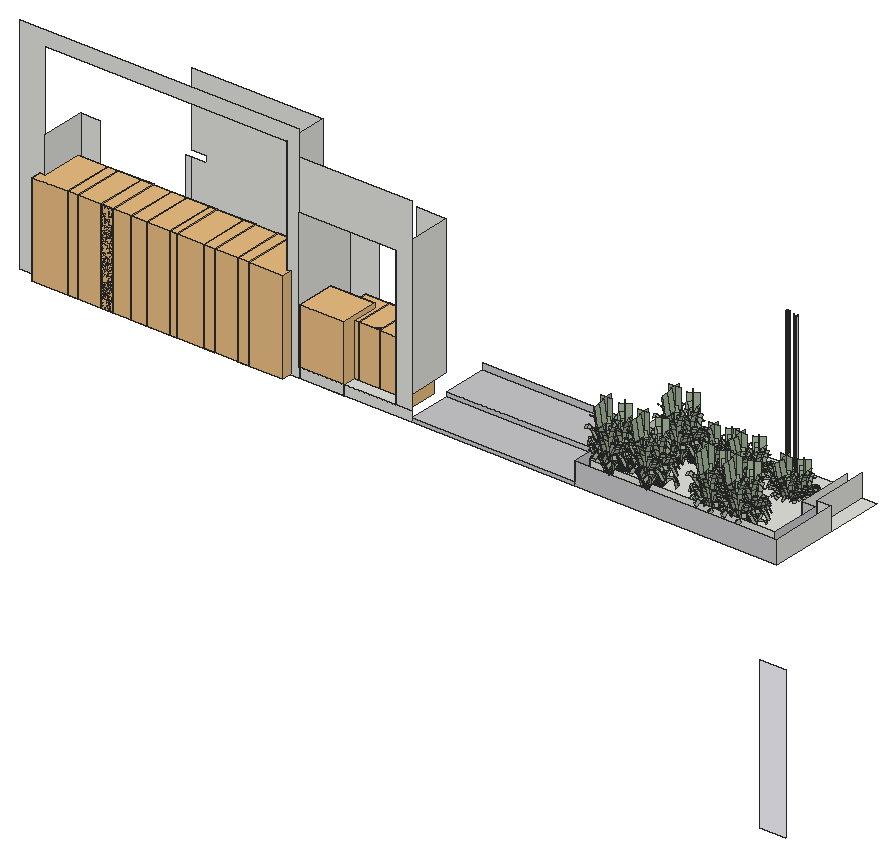
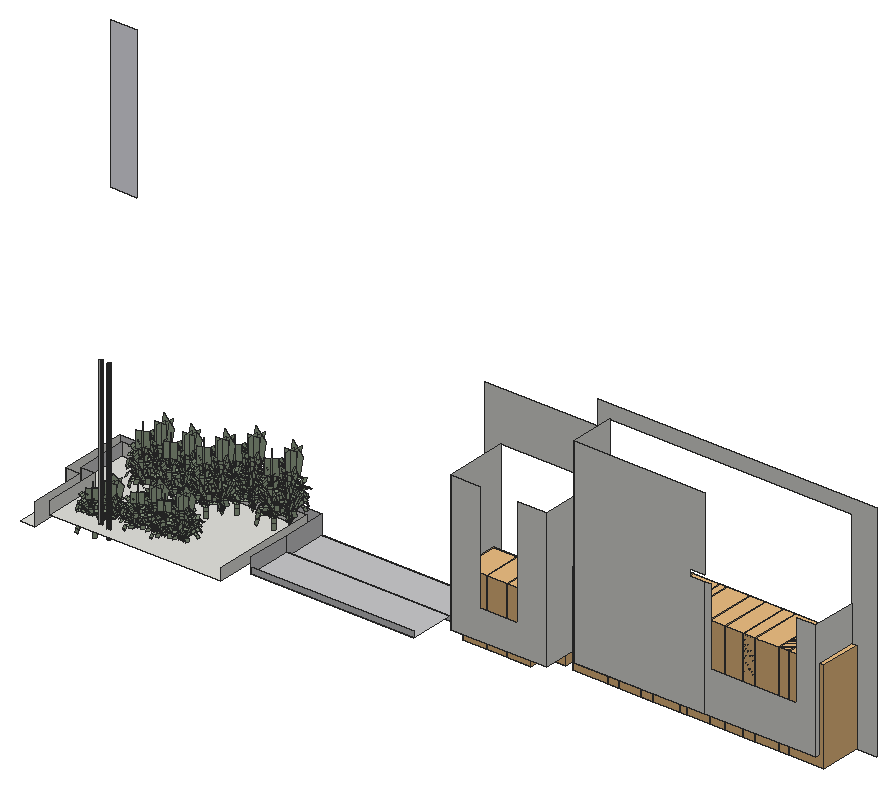
# SketchUp Ruby script. Lengths in inches.
U = 1.inch
M = Sketchup.active_model
def pt(a) = Geom::Point3d.new(a.map { |v| v * U })
def face(e, loops, mat)
  f = e.add_face(loops[0].map { |a| pt(a) })
  loops[1..].each { |l| e.add_face(l.map { |a| pt(a) }).erase! }
  f.material = f.back_material = mat if mat
  f
end
# faces: each face lists its corners as indices into pts; further lists are holes
def faces(e, pts, list, mat = nil) = list.each { |f| face(e, (f[0].is_a?(Array) ? f : [f]).map { |l| l.map { |i| pts[i] } }, mat) }
# xy, xz, yz: faces in a plane at the given z, y or x. An outline is a flat list of corners, or four numbers for a rectangle; further outlines are holes
def ring(l) = l.size == 4 ? [[l[0], l[1]], [l[2], l[1]], [l[2], l[3]], [l[0], l[3]]] : l.each_slice(2).to_a
def flat(e, list, mat, &to3) = list.each { |f| face(e, (f[0].is_a?(Array) ? f : [f]).map { |l| ring(l).map { |u, v| to3.(u, v) } }, mat) }
def xy(e, z, list, mat = nil) = flat(e, list, mat) { |x, y| [x, y, z] }
def xz(e, y, list, mat = nil) = flat(e, list, mat) { |x, z| [x, y, z] }
def yz(e, x, list, mat = nil) = flat(e, list, mat) { |y, z| [x, y, z] }
def lines(e, pts, list) = list.each { |a, b| e.add_line(pt(pts[a]), pt(pts[b])) }
# prism: a flat outline (further loops are holes) pulled along v
def prism(e, loops, v, mat = nil)
  f = face(e, loops, mat); d = Geom::Vector3d.new(v.map { |x| x * U })
  f.pushpull(f.normal.samedirection?(d) ? d.length : -d.length)
end
def box(e, o, s, mat = nil) = prism(e, [[o, [o[0] + s[0], o[1], o[2]], [o[0] + s[0], o[1] + s[1], o[2]], [o[0], o[1] + s[1], o[2]]]], [0, 0, s[2]], mat)
def at(x, y, z, deg = 0) = Geom::Transformation.translation(pt([x, y, z])) * Geom::Transformation.rotation(ORIGIN, Z_AXIS, deg.degrees)
def axes(o, x, y, z) = Geom::Transformation.new([*x, 0, *y, 0, *z, 0, *pt(o).to_a, 1])
def part(name) = M.definitions.add(name)
# library, detail: a bought-in or finely detailed component or shape, given as its bounding box
def library(name, o, s) = part(name).tap { |d| box(d.entities, o, s) }
def detail(e, o, s) = box(e.add_group.entities, o, s)
def put(e, d, t, mat = nil) = e.add_instance(d, t).tap { |i| i.material = mat if mat }
def group(e, t, mat = nil) = e.add_group.tap { |g| g.transformation = t; g.material = mat if mat }.entities
root = M.entities
M.materials.add("[0117_GhostWhite]").color = [248, 248, 255]
M.materials.add("[Polished Concrete New]").color = [200, 200, 203]
M.materials.add("hymenocallis littoralis").color = [156, 172, 146]
c1 = part("Group\#856")
xy(c1.entities,7.38,[[0,0,5.5,15.91]],"hymenocallis littoralis")
p = [[5.5,28.78,0],[5.5,26.79,3.44],[0,26.79,3.44],[0,28.78,0],[0,23.75,6],[5.5,23.75,6],
  [0,15.91,7.38],[5.5,15.91,7.38]]
faces(c1.entities,p,[[0,1,2,3],[4,2,1,5],[6,4,5,7]],"hymenocallis littoralis")
c2 = part("Group\#854")
xy(c2.entities,7.38,[[0,0,5.5,15.91],[0,15.91,5.5,23.87]],"hymenocallis littoralis")
p = [[5.5,31.07,4.3],[5.5,27.74,6.47],[0,27.74,6.47],[0,31.07,4.3],[0,23.87,7.38],[5.5,23.87,7.38]]
faces(c2.entities,p,[[0,1,2,3],[4,2,1,5]],"hymenocallis littoralis")
c3 = part("Group\#857")
xy(c3.entities,7.38,[[0,0,5.6,15.91]],"hymenocallis littoralis")
p = [[5.6,28.78,0],[5.6,26.79,3.44],[0,26.79,3.44],[0,28.78,0],[0,23.75,6],[5.6,23.75,6],
  [0,15.91,7.38],[5.6,15.91,7.38]]
faces(c3.entities,p,[[0,1,2,3],[4,2,1,5],[6,4,5,7]],"hymenocallis littoralis")
c4 = part("Group\#855")
put(c4.entities,c2,axes([6.09,8.57,-0.52],[0.446,0.85617,0.26089],[-0.18444,-0.19731,0.96283],[0.87582,-0.47754,0.0699]))
put(c4.entities,c2,axes([6.29,7.28,-1.71],[0.37058,0.92707,-0.05667],[-0.32382,0.19004,0.99128],[0.87712,-0.32925,0.34964]))
put(c4.entities,c2,axes([11.04,16.14,-0.7],[1,0,0],[0,0.16628,1.02662],[0,-1.18456,0.19186]))
c5 = part("Group\#860")
put(c5.entities,c1,axes([24.57,32.05,-1.76],[0.9552,-0.22102,-0.19681],[0.4036,0.95545,0.88585],[-0.00568,-0.67859,0.7345]))
put(c5.entities,c1,axes([23.95,29.24,-2.4],[0,1,0],[-0.76041,0,0.64945],[0.64945,0,0.76041]))
put(c5.entities,c1,axes([24.22,24.72,-0.48],[-0.70711,0.70711,0],[-0.32757,-0.32757,0.80237],[0.61237,0.61237,0.5]))
put(c5.entities,c2,axes([20.66,37.22,-0.63],[1.12361,0.03262,0.39091],[-0.43499,0.29739,0.78777],[0.09852,-1.27434,0.37535]))
put(c5.entities,c1,axes([28.75,24.45,-2.4],[-1,0,0],[0,-0.76041,0.64945],[0,0.64945,0.76041]))
put(c5.entities,c3,axes([30.4,30.98,-3.7],[0.65676,-0.72002,0.22414],[0.55667,0.66341,0.5],[-0.50871,-0.20361,0.83652]))
put(c5.entities,c3,axes([32.41,29.61,-3.7],[0.04029,-0.97372,0.22414],[0.85287,0.15038,0.5],[-0.52057,0.17102,0.83652]))
put(c5.entities,c1,axes([31.89,25.85,-1.76],[-0.92056,0.33739,-0.19681],[-0.5186,-0.89824,0.88585],[0.08952,0.67268,0.7345]))
put(c5.entities,c1,axes([25.55,34.78,-0.48],[0.86603,0.5,0],[-0.25,0.43301,0.86603],[0.43301,-0.75,0.5]))
put(c5.entities,c3,axes([20.4,16.9375,-8.07],[-0.70711,0.70711,0],[-0.35754,-0.35754,0.65422],[1.3987,1.3987,1.52882]))
put(c5.entities,c1,axes([32.86,34.14,-0.48],[0.76604,-0.64279,0],[0.32139,0.38302,0.86603],[-0.55667,-0.66341,0.5]))
put(c5.entities,c1,axes([27.15,34.7,-0.1],[0.82472,-0.17528,-0.53769],[0.53769,0.53769,0.64945],[0.17528,-0.82472,0.53769]))
put(c5.entities,c1,axes([33.58,28.77,-2.4],[0,-1,0],[0.76041,0,0.64945],[-0.64945,0,0.76041]))
put(c5.entities,c1,axes([26.43,23.87,-2.81],[-0.75126,0.04415,0.65853],[0.53769,-0.53769,0.64945],[0.38276,0.84199,0.3802]))
put(c5.entities,c1,axes([28.78,23.98,-2.4],[-1,0,0],[0,-0.76041,0.64945],[0,0.64945,0.76041]))
put(c5.entities,c1,axes([25.39,25.38,-2.4],[-0.70711,0.70711,0],[-0.53769,-0.53769,0.64945],[0.45923,0.45923,0.76041]))
put(c5.entities,c1,axes([27.32,21.63,-0.1],[-0.45923,0.70711,-0.53769],[-0.76041,0,0.64945],[0.45923,0.70711,0.53769]))
put(c5.entities,c1,axes([25.17,27.625,-1.76],[0.56416,0.80187,-0.19681],[-0.66673,0.66673,0.80532],[0.62659,-0.26057,0.7345]))
put(c5.entities,c3,axes([27.59,27.04,-3.96],[-0.8993,-0.06127,0.43301],[0.2962,-0.8138,0.5],[0.32175,0.57791,0.75]))
put(c5.entities,c3,axes([26.98,24.5,-3.18],[-0.5,0.86603,0],[-0.75,-0.43301,0.5],[0.43301,0.25,0.86603]))
put(c5.entities,c3,axes([24.55,27.74,-3.7],[0.29517,0.92878,0.22414],[-0.85287,0.15038,0.5],[0.43068,-0.33875,0.83652]))
put(c5.entities,c3,axes([24.26,29.8,-3.18],[0.76604,0.64279,0],[-0.47317,0.5639,0.425],[0.32139,-0.38302,0.86603]))
put(c5.entities,c3,axes([25.98,32.46,-3.18],[1,0,0],[0,0.86603,0.5],[0,-0.5,0.86603]))
put(c5.entities,c1,axes([28.78,33.57,-2.4],[1,0,0],[0,0.76041,0.64945],[0,-0.64945,0.76041]))
put(c5.entities,c4,at(14.99,21.38,2.5))
put(c5.entities,c2,axes([34.63,26.34,-1.46],[-0.70089,-0.70877,0.07994],[0.4756,-0.38088,0.79293],[-0.53156,0.59378,0.60405]))
put(c5.entities,c2,axes([28.14,16.92,1.8125],[-1.19719,0.6912,0],[-0.09607,-0.16641,0.94244],[0.68444,1.18549,0.17613]))
put(c5.entities,c2,axes([31.5625,35.84,0.97],[0.66765,-1.1564,0.35779],[0.04445,0.30732,0.91033],[-1.20828,-0.64496,0.17012]))
put(c5.entities,c2,axes([38.94,22.51,0.89],[-0.97932,-0.67164,-0.05202],[0.27787,-0.41401,0.90999],[-0.85985,0.93577,0.32097]))
put(c5.entities,c2,axes([38.44,21.09,1.98],[-1.02864,-0.54856,0.2395],[0.33481,0.06999,0.88388],[-0.77261,1.08328,0.06417]))
put(c5.entities,c3,axes([35.02,30.51,-1.3],[-0.17365,-0.98481,0],[0.60224,-0.10619,0.79122],[-0.7792,0.13739,0.61153]))
put(c5.entities,c3,axes([29.41,22.33,-1.3],[-0.93969,0.34202,0],[-0.20915,-0.57465,0.79122],[0.27061,0.74351,0.61153]))
put(c5.entities,c2,axes([19.64,36,-1.62],[1.18194,0.09546,0.08234],[-0.14377,0.68823,0.76313],[0.21457,-1.1326,0.62386]))
put(c5.entities,c3,axes([24.25,24.14,-1.3],[-0.34202,0.93969,0],[-0.57465,-0.20915,0.79122],[0.74351,0.27061,0.61153]))
put(c5.entities,c3,axes([25.98,34.61,-1.3],[1,0,0],[0,0.61153,0.79122],[0,-0.79122,0.61153]))
put(c5.entities,c3,axes([31.16,34.41,-1.64],[0.56518,-0.80224,-0.19234],[0.73413,0.34233,0.72935],[-0.47639,-0.50772,0.71782]))
put(c5.entities,c3,axes([40.52,26.84,-5.82],[-0.42262,-0.90631,0],[0.48019,-0.22391,0.68552],[-1.43418,0.66877,1.22305]))
put(c5.entities,c1,axes([29.86,38.42,-1.01],[0.89064,-0.37013,0.26413],[-0.03924,0.63286,1.01918],[-0.45353,-0.76487,0.45748]))
put(c5.entities,c1,axes([29.34,22.4,-0.48],[-0.99619,-0.08716,0],[0.04358,-0.4981,0.86603],[-0.07548,0.86273,0.5]))
c6 = part("Group\#858")
xz(c6.entities,10.07,[[9.07,0,10.07,31.01],[0,31.01,0,45.12,20.13,45.12,20.13,31.01,10.07,31.01,10.07,32.58,9.07,32.58,9.07,31.01]],"hymenocallis littoralis")
yz(c6.entities,10.07,[[0,31.01,20.13,45.12]],"hymenocallis littoralis")
p = [[9.57,9.2,0],[10.07,10.07,0],[10.07,10.07,31.01],[10.07,10.07,32.58],[9.57,9.2,32.58]]
faces(c6.entities,p,[[0,1,2,3,4]],"hymenocallis littoralis")
c7 = part("cây lá nắng")
put(c7.entities,c5,axes([49.26,-2.75,0],[0.63109,0.63109,0],[-0.63109,0.63109,0],[0,0,0.935]))
g1 = group(c7.entities,at(26.6,-8.68,0))
put(g1,c1,axes([-4.72,35.73,-1.65],[0.74231,0.46334,-0.18402],[-0.34827,0.85768,0.82827],[0.42467,-0.43184,0.68675]))
put(g1,c1,axes([-3.34,33.57,-2.24],[-0.63109,0.63109,0],[-0.47989,-0.47989,0.60723],[0.40986,0.40986,0.71098]))
put(g1,c1,axes([-0.3125,30.89,-0.45],[-0.8925,0,0],[0,-0.41345,0.75022],[0,0.77293,0.4675]))
put(g1,c2,axes([-10.79,39.66,-0.59],[0.68852,0.72969,0.3655],[-0.4622,-0.08684,0.73657],[0.86641,-0.74205,0.35095]))
put(g1,c1,axes([2.71,33.57,-2.24],[-0.63109,-0.63109,0],[0.47989,-0.47989,0.60723],[-0.40986,0.40986,0.71098]))
put(g1,c3,axes([-0.37,38.74,-3.46],[0.86887,-0.03992,0.20957],[-0.06737,0.76999,0.4675],[-0.19255,-0.44954,0.78214]))
put(g1,c3,axes([1.76,39.14,-3.46],[0.63993,-0.58908,0.20957],[0.44333,0.63315,0.4675],[-0.43646,-0.2206,0.78214]))
put(g1,c1,axes([3.81,36.4375,-1.65],[-0.79389,-0.36803,-0.18402],[0.23959,-0.89415,0.82827],[-0.36803,0.48102,0.68675]))
put(g1,c1,axes([-5.83,38.07,-0.45],[0.231,0.86209,0],[-0.43104,0.1155,0.80973],[0.74659,-0.20005,0.4675]))
put(g1,c3,axes([2.18,23.5625,-7.55],[-0.8925,0,0],[0,-0.45128,0.6117],[0,1.76542,1.42944]))
put(g1,c1,axes([-0.8125,42.28,-0.45],[0.8891,0.07779,0],[-0.03889,0.44455,0.80973],[0.06737,-0.76999,0.4675]))
put(g1,c1,axes([-4.76,39.03,-0.09],[0.63109,0.40986,-0.50274],[0,0.67866,0.60723],[0.63109,-0.40986,0.50274]))
put(g1,c1,axes([3.03,39.35,-2.24],[0.63109,-0.63109,0],[0.47989,0.47989,0.60723],[-0.40986,-0.40986,0.71098]))
put(g1,c1,axes([1.61,31.74,-2.625],[-0.50198,-0.44625,0.61573],[0.67866,0,0.60723],[-0.28982,0.77293,0.35549]))
put(g1,c1,axes([3.03,33.3,-2.24],[-0.63109,-0.63109,0],[0.47989,-0.47989,0.60723],[-0.40986,0.40986,0.71098]))
put(g1,c1,axes([0.01,32.04,-2.24],[-0.8925,0,0],[0,-0.67866,0.60723],[0,0.57963,0.71098]))
put(g1,c1,axes([3.59,30.89,-0.09],[-0.73607,0.15643,-0.50274],[-0.47989,-0.47989,0.60723],[-0.15643,0.73607,0.50274]))
put(g1,c1,axes([-1.55,33.32,-1.65],[-0.15002,0.86209,-0.18402],[-0.84154,0,0.75297],[0.55988,0.231,0.68675]))
put(g1,c3,axes([0.35,34.48,-3.71],[-0.52887,-0.60621,0.40487],[0.70051,-0.32665,0.4675],[-0.16166,0.56777,0.70125]))
put(g1,c3,axes([2.61,39.13,-1.74],[-0.86209,0.231,0],[-0.23031,-0.85954,0.15531],[0.03162,0.11799,0.91645]))
put(g1,c3,axes([-2.02,33,-3.46],[-0.39986,0.77243,0.20957],[-0.63315,-0.44333,0.4675],[0.48558,0.05802,0.78214]))
put(g1,c3,axes([-3.49,34.12,-2.97],[0.07779,0.8891,0],[-0.65449,0.05726,0.39737],[0.44455,-0.03889,0.80973]))
put(g1,c3,axes([-4.09,36.88,-2.97],[0.63109,0.63109,0],[-0.54654,0.54654,0.4675],[0.31555,-0.31555,0.80973]))
put(g1,c1,axes([-3.02,39.35,-2.24],[0.63109,0.63109,0],[-0.47989,0.47989,0.60723],[0.40986,-0.40986,0.71098]))
put(g1,c4,axes([-4.03,22.95,2.33],[0.63109,0.63109,0],[-0.63109,0.63109,0],[0,0,0.935]))
put(g1,c2,axes([5.24,38.48,-1.37],[0.00497,-0.88963,0.07474],[0.54052,0.05978,0.74139],[-0.71019,0.03927,0.56479]))
put(g1,c2,axes([7.08,28.4375,1.7],[-1.19175,-0.31933,0],[0.04439,-0.16565,0.88118],[-0.31621,1.1801,0.16468]))
put(g1,c2,axes([-2.7,42.54,0.91],[1.15114,-0.30845,0.33454],[-0.1659,0.22199,0.85115],[-0.3555,-1.16957,0.15907]))
put(g1,c2,axes([10.37,38.78,0.83],[-0.19417,-1.04191,-0.04864],[0.43664,-0.08592,0.85084],[-1.1332,0.04791,0.30011]))
put(g1,c2,axes([10.95,37.5625,1.85],[-0.30298,-0.99536,0.22393],[0.16713,0.25547,0.82643],[-1.17124,0.19607,0.06]))
put(g1,c3,axes([2.84,41.36,-1.22],[0.51192,-0.73109,0],[0.44708,0.31305,0.73979],[-0.57846,-0.40504,0.57178]))
put(g1,c3,axes([4.47,32.65,-1.22],[-0.80888,-0.37719,0],[0.23066,-0.49465,0.73979],[-0.29844,0.64,0.57178]))
put(g1,c2,axes([-10.32,35.12,-1.51],[0.68567,0.80616,0.07699],[-0.52507,0.3436,0.71352],[0.85019,-0.57936,0.58331]))
put(g1,c3,axes([0.07,30.54,-1.22],[-0.80888,0.37719,0],[-0.23066,-0.49465,0.73979],[0.29844,0.64,0.57178]))
put(g1,c3,axes([-5.45,38.24,-1.22],[0.63109,0.63109,0],[-0.38593,0.38593,0.73979],[0.49934,-0.49934,0.57178]))
put(g1,c3,axes([-2.05,41.38,-1.53],[0.86296,-0.14961,-0.17984],[0.24726,0.67935,0.68194],[0.01977,-0.62107,0.67116]))
put(g1,c3,axes([8.63,42.51,-5.4375],[0.30525,-0.83868,0],[0.44435,0.16173,0.64096],[-1.32716,-0.48305,1.14356]))
put(g1,c1,axes([-5.4,43.09,-0.94],[0.79566,0.32849,0.24696],[-0.42416,0.37462,0.95293],[0.19648,-0.76892,0.42774]))
put(g1,c1,axes([4.38,32.65,-0.45],[-0.57369,-0.68369,0],[0.34185,-0.28684,0.80973],[-0.5921,0.49683,0.4675]))
put(g1,c3,axes([-2,33.84,-0.15],[-0.24601,0.85793,0],[-0.85539,-0.24528,0.15531],[0.11742,0.03367,0.91645]))
put(g1,c3,axes([0.17,30.83,-4.47],[-0.24601,0.85793,0],[-0.85539,-0.24528,0.15531],[0.11742,0.03367,0.91645]))
put(g1,c3,axes([-1.97,32.18,-4.47],[0.58524,0.67383,0],[-0.67184,0.58351,0.15531],[0.09222,-0.0801,0.91645]))
put(g1,c3,axes([-2,34.71,-4.47],[0.88392,-0.12346,0],[0.12309,0.88131,0.15531],[-0.0169,-0.12098,0.91645]))
put(g1,c3,axes([0.11,36.12,-4.47],[0.37822,-0.8084,0],[0.80601,0.37711,0.15531],[-0.11064,-0.05177,0.91645]))
put(c7.entities,c6,axes([29.71,14.29,6.94],[0.425,0.73612,0],[-0.6771,0.39092,-0.33349],[-0.26859,0.15507,0.72712]))
put(c7.entities,c6,axes([42.0625,26.12,6.94],[0.85,0,0],[0,0.78185,-0.33349],[0,0.33349,0.78185]))
put(c7.entities,c5,axes([7.3125,23.0625,0],[0.8925,0,0],[0,0.8925,0],[0,0,0.935]))
put(c7.entities,c6,axes([24.4375,40.23,2.05],[0.85,0,0],[0,0.85,0],[0,0,0.85]))
c8 = part("Planting+101")
put(c8.entities,c7,axes([21.34,32.96,-4.59],[0,-0.71,0],[-0.71,0,0],[0,0,0.71]))
c9 = library("Potted plant",[-6.35,-9.74,0],[57.68,49.85,85.16])
xy(root,0,[[1425.51,521.59,1443.95,594.47]])
xy(root,4.5,[[971.9,433.09,1182.84,490.26]],"[Polished Concrete New]")
xy(root,10.3125,[[971.9,490.26,1182.84,547.43]],"[Polished Concrete New]")
xy(root,12.91,[[497.32,433.09,810.8,490.53],[825.44,433.09,950.63,515.34]])
xy(root,13.1875,[[[1193.75,444.01,1433.03,444.01,1433.03,510.68,1414.59,510.68,1414.59,583.56,1193.75,583.56],[1361.93,564.77,1361.35,564.82,1360.8,565.01,1360.3125,565.34,1359.93,565.78,1359.67,566.31,1359.5625,566.88,1359.6,567.47,1359.8,568.02,1360.125,568.51,1360.57,568.89,1361.1,569.15,1361.67,569.26,1362.26,569.22,1362.8125,569.02,1363.3,568.69,1363.68,568.25,1363.94,567.72,1364.05,567.15,1364,566.5625,1363.8125,566.01,1363.48,565.52,1363.04,565.14,1362.51,564.88]]])
xz(root,0,[[1769.06,0,1802.44,193.9375]],"[0117_GhostWhite]")
xz(root,433.09,[[[465.27,0,825.44,287.9375],[497.32,12.91,810.8,269.5625]],[825.44,0,971.9,12.91],[950.63,12.91,971.9,12.91,971.9,256.3125,825.44,256.3125,825.44,191.73,950.63,191.73]])
xz(root,433.09,[[971.9,0,1182.84,4.5],[1182.84,0,1443.95,29.3125]],"[Polished Concrete New]")
xz(root,444.01,[[1193.75,13.1875,1433.03,29.3125]])
xz(root,490.26,[[971.9,4.5,1182.84,10.3125]],"[Polished Concrete New]")
xz(root,490.53,[[497.32,12.91,640.85,12.91,640.85,166.1,633.9,166.1,633.9,67.73,522.65,67.73,522.65,166.1,497.32,166.1],[640.85,12.91,810.8,12.91,810.8,269.5625,640.85,269.5625,640.85,174.17,660.32,174.17,660.32,166.1,640.85,166.1]])
xz(root,510.68,[[1414.59,13.1875,1433.03,29.3125]],"[Polished Concrete New]")
xz(root,515.34,[[825.44,12.91,950.63,12.91,950.63,191.73,912.07,191.73,912.07,51.84,862.83,51.84,862.83,191.73,825.44,191.73]])
xz(root,521.59,[[1425.51,0,1443.95,29.3125]])
xz(root,547.43,[[971.9,10.3125,1182.84,18.375]],"[Polished Concrete New]")
yz(root,497.32,[[433.09,12.91,490.53,166.1]])
yz(root,810.8,[[433.09,12.91,490.53,269.5625]])
yz(root,825.44,[[433.09,12.91,515.34,191.73]])
yz(root,950.63,[[433.09,12.91,515.34,191.73]])
yz(root,1182.84,[[433.09,4.5,490.26,29.3125],[490.26,10.3125,547.43,29.3125]],"[Polished Concrete New]")
yz(root,1193.75,[[444.01,13.1875,583.56,29.3125]])
yz(root,1414.59,[[510.68,13.1875,583.56,29.3125]])
yz(root,1425.51,[[521.59,0,594.47,29.3125]])
yz(root,1433.03,[[444.01,13.1875,510.68,29.3125]],"[Polished Concrete New]")
yz(root,1443.95,[[433.09,0,521.59,29.3125]])
p = [[1350.05,565.01,0],[1350.6,564.82,0],[1350.6,564.82,202.53],[1350.05,565.01,202.53],[1351.18,564.77,0],[1351.18,564.77,202.53],
  [1351.76,564.88,0],[1351.76,564.88,202.53],[1352.29,565.14,0],[1352.29,565.14,202.53],[1349.5625,565.34,0],[1349.5625,565.34,202.53],
  [1352.73,565.52,0],[1352.73,565.52,202.53],[1349.18,565.78,0],[1349.18,565.78,202.53],[1353.0625,566.01,0],[1353.0625,566.01,202.53],
  [1348.92,566.31,0],[1348.92,566.31,202.53],[1353.25,566.5625,0],[1353.25,566.5625,202.53],[1348.8125,566.88,0],[1348.8125,566.88,202.53],
  [1353.3,567.15,0],[1353.3,567.15,202.53],[1348.85,567.47,0],[1348.85,567.47,202.53],[1353.19,567.72,0],[1353.19,567.72,202.53],
  [1349.05,568.02,0],[1349.05,568.02,202.53],[1352.93,568.25,0],[1352.93,568.25,202.53],[1349.375,568.51,0],[1349.375,568.51,202.53],
  [1352.55,568.69,0],[1352.55,568.69,202.53],[1349.82,568.89,0],[1349.82,568.89,202.53],[1352.0625,569.02,0],[1352.0625,569.02,202.53],
  [1350.35,569.15,0],[1350.35,569.15,202.53],[1351.51,569.22,0],[1351.51,569.22,202.53],[1350.92,569.26,0],[1350.92,569.26,202.53],
  [1360.8,565.01,202.53],[1360.8,565.01,13.1875],[1361.35,564.82,13.1875],[1361.35,564.82,202.53],[1361.93,564.77,13.1875],[1361.93,564.77,202.53],
  [1362.51,564.88,13.1875],[1362.51,564.88,202.53],[1363.04,565.14,13.1875],[1363.04,565.14,202.53],[1360.3125,565.34,202.53],[1360.3125,565.34,13.1875],
  [1363.48,565.52,13.1875],[1363.48,565.52,202.53],[1359.93,565.78,202.53],[1359.93,565.78,13.1875],[1363.8125,566.01,13.1875],[1363.8125,566.01,202.53],
  [1359.67,566.31,202.53],[1359.67,566.31,13.1875],[1364,566.5625,13.1875],[1364,566.5625,202.53],[1359.5625,566.88,202.53],[1359.5625,566.88,13.1875],
  [1364.05,567.15,13.1875],[1364.05,567.15,202.53],[1361.8,567.02,203.98],[1361.8,567.02,0]]
faces(root,p,[[0,1,2,3],[1,4,5,2],[4,6,7,5],[6,8,9,7],[10,0,3,11],[8,12,13,9],[14,10,11,15],[12,16,17,13],
  [18,14,15,19],[16,20,21,17],[22,18,19,23],[20,24,25,21],[26,22,23,27],[24,28,29,25],[30,26,27,31],[28,32,33,29],
  [34,30,31,35],[32,36,37,33],[38,34,35,39],[36,40,41,37],[42,38,39,43],[40,44,45,41],[46,42,43,47],[44,46,47,45],
  [48,49,50,51],[51,50,52,53],[53,52,54,55],[55,54,56,57],[58,59,49,48],[57,56,60,61],[62,63,59,58],[61,60,64,65],
  [66,67,63,62],[65,64,68,69],[70,71,67,66],[69,68,72,73]])
lines(root,p,[[74,75]])
put(root,c8,axes([1223.54,444.01,31.06],[1.18,0,0],[0,1,0],[0,0,3]))
put(root,c8,axes([1271.42,444.01,31.06],[1.18,0,0],[0,1,0],[0,0,3]))
put(root,c9,axes([718.72,433.26,0],[1.02147,0,0],[0,1.31,0],[0,0,1.41]))
put(root,c9,axes([625.25,433.26,0],[1.02147,0,0],[0,1.31,0],[0,0,1.41]))
put(root,c9,axes([674.8,433.26,0],[1.02147,0,0],[0,1.31,0],[0,0,1.41]))
put(root,c9,axes([497.32,433.26,0],[1.02147,0,0],[0,1.31,0],[0,0,1.41]))
put(root,c9,axes([762.96,433.26,0],[1.02147,0,0],[0,1.31,0],[0,0,1.41]))
put(root,c9,axes([586.18,433.26,0],[1.02147,0,0],[0,1.31,0],[0,0,1.41]))
put(root,c9,axes([542.9,433.26,0],[1.02147,0,0],[0,1.31,0],[0,0,1.41]))
put(root,c9,at(832.96,442.84,0))
put(root,c8,axes([1344.48,457.08,13.43],[1.18,0,0],[0,1,0],[0,0,3]))
put(root,c8,axes([1380.17,457.08,13.43],[1.18,0,0],[0,1,0],[0,0,3]))
put(root,c9,at(896.52,458.93,-5.18))
put(root,c9,at(865.77,458.93,-5.18))
put(root,c8,axes([1277.56,486.63,43.92],[1.18,0,0],[0,1,0],[0,0,3]))
put(root,c8,axes([1296.84,525.99,13.1875],[1.18,0,0],[0,1,0],[0,0,2]))
put(root,c8,axes([1328.76,529.58,13.1875],[1.18,0,0],[0,1,0],[0,0,2]))
put(root,c8,axes([1381.95,536.31,2.14],[1.18,0,0],[0,1,0],[0,0,2]))
